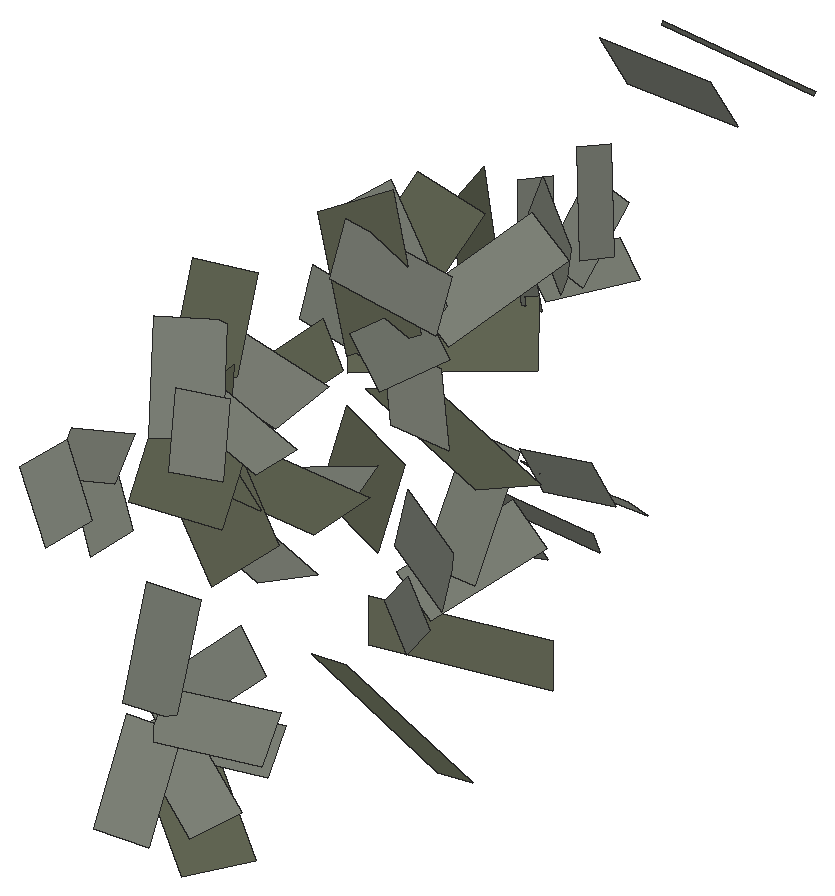
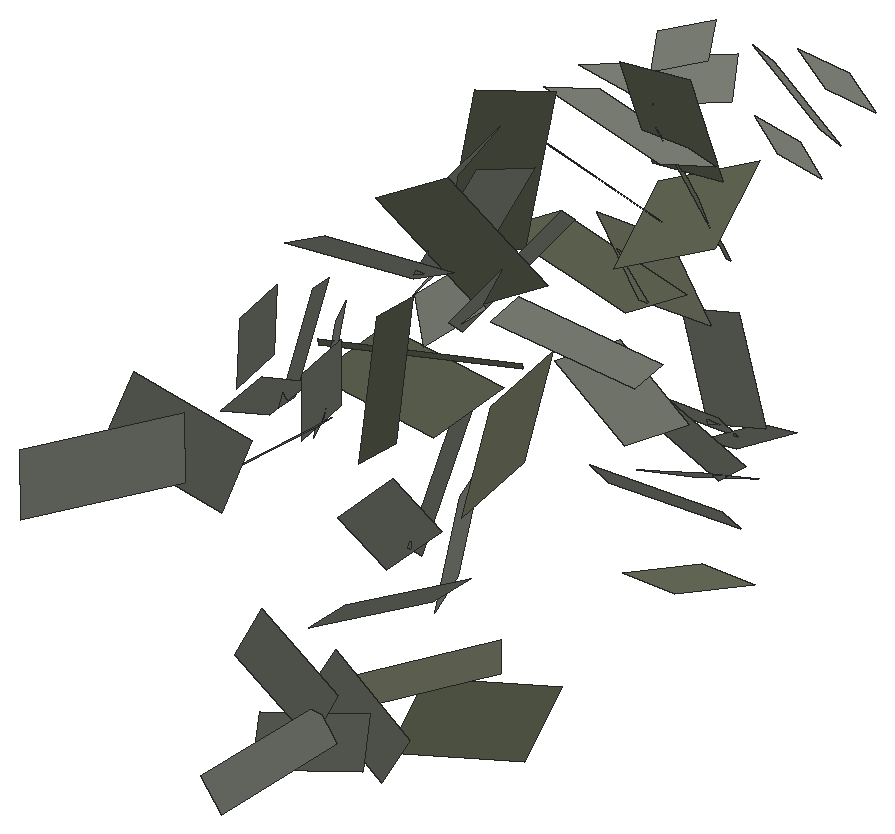
# SketchUp Ruby script. Lengths in inches.
U = 1.inch
M = Sketchup.active_model
def pt(a) = Geom::Point3d.new(a.map { |v| v * U })
def face(e, loops, mat)
  f = e.add_face(loops[0].map { |a| pt(a) })
  loops[1..].each { |l| e.add_face(l.map { |a| pt(a) }).erase! }
  f.material = f.back_material = mat if mat
  f
end
# faces: each face lists its corners as indices into pts; further lists are holes
def faces(e, pts, list, mat = nil) = list.each { |f| face(e, (f[0].is_a?(Array) ? f : [f]).map { |l| l.map { |i| pts[i] } }, mat) }
# xy, xz, yz: faces in a plane at the given z, y or x. An outline is a flat list of corners, or four numbers for a rectangle; further outlines are holes
def ring(l) = l.size == 4 ? [[l[0], l[1]], [l[2], l[1]], [l[2], l[3]], [l[0], l[3]]] : l.each_slice(2).to_a
def flat(e, list, mat, &to3) = list.each { |f| face(e, (f[0].is_a?(Array) ? f : [f]).map { |l| ring(l).map { |u, v| to3.(u, v) } }, mat) }
def xy(e, z, list, mat = nil) = flat(e, list, mat) { |x, y| [x, y, z] }
def xz(e, y, list, mat = nil) = flat(e, list, mat) { |x, z| [x, y, z] }
def yz(e, x, list, mat = nil) = flat(e, list, mat) { |y, z| [x, y, z] }
def lines(e, pts, list) = list.each { |a, b| e.add_line(pt(pts[a]), pt(pts[b])) }
# prism: a flat outline (further loops are holes) pulled along v
def prism(e, loops, v, mat = nil)
  f = face(e, loops, mat); d = Geom::Vector3d.new(v.map { |x| x * U })
  f.pushpull(f.normal.samedirection?(d) ? d.length : -d.length)
end
def box(e, o, s, mat = nil) = prism(e, [[o, [o[0] + s[0], o[1], o[2]], [o[0] + s[0], o[1] + s[1], o[2]], [o[0], o[1] + s[1], o[2]]]], [0, 0, s[2]], mat)
def at(x, y, z, deg = 0) = Geom::Transformation.translation(pt([x, y, z])) * Geom::Transformation.rotation(ORIGIN, Z_AXIS, deg.degrees)
def axes(o, x, y, z) = Geom::Transformation.new([*x, 0, *y, 0, *z, 0, *pt(o).to_a, 1])
def part(name) = M.definitions.add(name)
# library, detail: a bought-in or finely detailed component or shape, given as its bounding box
def library(name, o, s) = part(name).tap { |d| box(d.entities, o, s) }
def detail(e, o, s) = box(e.add_group.entities, o, s)
def put(e, d, t, mat = nil) = e.add_instance(d, t).tap { |i| i.material = mat if mat }
def group(e, t, mat = nil) = e.add_group.tap { |g| g.transformation = t; g.material = mat if mat }.entities
root = M.entities
M.materials.add("viburnumblaasdfas0df1w06d").color = [98, 102, 84]
M.materials.add("viburnumbladsadfasdfad0w122").color = [125, 129, 119]
c1 = part("Component\#314")
p = [[0.14,0,0],[2.58,0.05,0.25],[2.44,5.11,2.64],[0,5.05,2.39]]
faces(c1.entities,p,[[0,1,2,3]],"viburnumblaasdfas0df1w06d")
c2 = part("viburnumblad1\#2")
put(c2.entities,c1,axes([-37.25,6.23,19.31],[75.98784,0,0],[0,65.50676,0],[0,0,75.98784]))
c3 = part("Component\#315")
p = [[0.25,0,0],[2.05,0.01,0.35],[1.81,4.2,1.66],[0,4.19,1.3125]]
faces(c3.entities,p,[[0,1,2,3]],"viburnumbladsadfasdfad0w122")
c4 = part("viburnumblad2")
put(c4.entities,c3,axes([-19.23,-4.49,-32.18],[83.35428,0,0],[0,79.38502,0],[0,0,83.35428]))
put(root,c2,axes([2216.77,275.47,24.61],[-0.00255,0.011,0.00125],[-0.00551,-0.00279,0.01135],[0.00975,0.00148,0.00412]))
put(root,c4,axes([2215.32,257.68,28.24],[0.00143,-0.00635,-0.00868],[0.00992,-0.00012,0.00155],[-0.0013,-0.00861,0.00528]))
put(root,c4,axes([2215.7,277.85,15.48],[-0.00478,-0.00491,0.00751],[0.00915,-0.00588,0.00198],[0.00339,0.00769,0.00718]))
put(root,c2,axes([2216.48,261.41,27.22],[0.01164,0.00293,-0.00079],[-0.00215,0.01041,0.00877],[0.00216,-0.00738,0.00809]))
put(root,c4,axes([2216.16,256.38,28.67],[-0.00668,-0.00514,-0.00687],[0.00865,-0.00485,-0.0047],[-0.00103,-0.00803,0.00606]))
put(root,c4,axes([2216.17,258.49,27.46],[-0.00601,-0.0039,-0.00689],[0.00865,-0.00485,-0.0047],[-0.00175,-0.00854,0.00529]))
put(root,c2,axes([2216.23,265.53,26.16],[-0.01393,-0.0074,0.00333],[0.00558,-0.01491,-0.00981],[0.00654,-0.00631,0.01332]))
put(root,c4,axes([2215.15,286.03,28.11],[-0.00284,-0.00899,0.01128],[0.01228,-0.00546,-0.00125],[0.00539,0.01,0.00933]))
put(root,c2,axes([2215.12,262.56,25.59],[0.00605,-0.00776,-0.00693],[0.01168,0.0029,0.00677],[-0.00267,-0.00844,0.00676]))
put(root,c4,axes([2215.67,279.9375,17.63],[0.0086,-0.00684,0.0012],[0.00538,0.00535,-0.00804],[0.0044,0.00684,0.00749]))
put(root,c4,axes([2215.47,279.03,16.375],[0.00269,-0.008,0.00714],[0.0092,-0.00069,-0.00424],[0.00383,0.00759,0.00707]))
put(root,c4,axes([2215.8,266.32,21.68],[-0.0065,-0.01157,-0.00112],[0.01142,-0.00611,-0.00313],[0.00221,-0.00249,0.0129]))
put(root,c2,axes([2215.51,263.71,15.08],[-0.00788,-0.01001,-0.0014],[0.00865,-0.00529,-0.01087],[0.00682,-0.00657,0.00863]))
put(root,c4,axes([2216.59,258.75,18.54],[0.01026,0.00498,-0.00256],[-0.00015,0.00559,0.01026],[0.0056,-0.00897,0.00496]))
put(root,c4,axes([2218.89,269.98,25.88],[-0.00545,0.00916,0.00529],[-0.00808,-0.00821,0.00589],[0.00818,-0.00089,0.00998]))
put(root,c2,axes([2216.46,272.24,21.13],[-0.00936,-0.00465,0.0096],[0.00338,-0.01554,-0.00424],[0.01026,-0.00044,0.00979]))
put(root,c4,axes([2218.34,276.4,26.26],[-0.00065,0.00993,-0.00423],[-0.00522,0.0028,0.00703],[0.00831,0.00266,0.0042]))
put(root,c4,axes([2215.34,287.43,29.63],[0.00691,-0.01139,0.00621],[0.0117,0.00243,-0.00856],[0.0056,0.00897,0.01021]))
put(root,c2,axes([2214.76,271.4,13.64],[0.00066,-0.01186,0.00699],[0.01121,-0.00532,-0.01007],[0.0098,0.00532,0.0081]))
put(root,c4,axes([2215.58,266.09,23.5],[0.00323,-0.01225,-0.0041],[0.01276,0.00369,-0.00099],[0.00204,-0.00369,0.01263]))
put(root,c2,axes([2216.34,269.37,27.16],[0.01029,0.00428,-0.00658],[0.00078,0.01194,0.00879],[0.00737,-0.00649,0.00685]))
put(root,c4,axes([2217.47,262.76,30.71],[-0.01238,-0.00774,-0.00167],[0.00772,-0.01057,-0.00819],[0.00296,-0.0074,0.01235]))
put(root,c4,axes([2216.15,260.25,18.125],[0.00784,-0.00117,-0.00859],[0.00729,0.00715,0.00568],[0.00468,-0.00917,0.00553]))
put(root,c4,axes([2218.99,269.42,27.52],[0.00288,0.01252,0.00147],[-0.00904,0.00098,0.00938],[0.00888,-0.00309,0.00888]))
put(root,c4,axes([2215.99,261.56,17.28],[0.00079,-0.00637,-0.0092],[0.01172,0.00425,-0.00193],[0.00425,-0.00877,0.00644]))
put(root,c4,axes([2218.42,259.42,17.8],[-0.01026,-0.00498,0.00256],[0.0015,-0.00759,-0.00876],[0.0054,-0.00736,0.0073]))
put(root,c2,axes([2215.96,263.29,26.33],[0.00918,-0.00623,-0.00469],[0.00881,0.01006,0.00379],[0.00131,-0.00544,0.00952]))
put(root,c4,axes([2216.91,279.56,17.11],[-0.0048,-0.00448,0.0089],[0.00915,-0.00588,0.00198],[0.00393,0.00822,0.00626]))
put(root,c2,axes([2215.07,271.54,26.12],[0.00626,-0.00918,-0.00848],[0.01094,0.01129,-0.00412],[0.00772,-0.00395,0.00939]))
put(root,c2,axes([2216.52,264.34,24.43],[-0.00713,-0.00827,-0.00706],[0.01264,-0.00623,-0.00545],[-0.00006,-0.00799,0.0088]))
put(root,c4,axes([2217.31,260.76,17.73],[-0.00667,-0.00821,-0.00496],[0.00888,-0.00228,-0.00816],[0.00454,-0.00802,0.00718]))
put(root,c4,axes([2216.21,264.04,29.79],[-0.0037,-0.01142,-0.00741],[0.01514,-0.00214,-0.00425],[0.00214,-0.0084,0.01187]))
put(root,c4,axes([2217.89,277.41,26.43],[0.00544,-0.00271,-0.00718],[0.0003,0.00981,-0.00339],[0.00825,0.00152,0.00476]))
put(root,c2,axes([2218.31,268.12,27.22],[0.00679,0.01089,0.00142],[-0.00667,0.00218,0.0129],[0.00902,-0.00665,0.00468]))
put(root,c2,axes([2215.76,271.5,16],[0.00753,-0.01126,-0.00255],[0.00884,0.00827,-0.01044],[0.00867,0.00351,0.01012]))
put(root,c4,axes([2218.02,270.95,18.42],[0.00716,-0.00025,-0.0097],[-0.0002,0.01356,-0.00049],[0.01011,0.00042,0.00745]))
put(root,c4,axes([2218.97,276.95,27.07],[0.00435,0.00477,-0.00798],[-0.00392,0.00825,0.00263],[0.00812,0.00193,0.0048]))
put(root,c4,axes([2218.92,276.9,25.2],[-0.0065,0.00265,0.00695],[0.00166,-0.0098,0.00501],[0.00741,0.00415,0.00458]))
put(root,c4,axes([2219.77,276.72,26.18],[-0.00523,0.00868,0.00226],[-0.00357,-0.00459,0.00897],[0.00802,0.00357,0.00411]))
put(root,c2,axes([2216.41,264.9,24.47],[-0.00228,-0.0125,-0.00287],[0.01428,-0.00152,-0.00471],[0.00336,-0.00314,0.01093]))
put(root,c4,axes([2219.37,270.55,19.34],[0.00427,0.00859,-0.00811],[-0.005,0.00913,0.00703],[0.0107,0.00084,0.00653]))
put(root,c4,axes([2220.65,269.3125,28.34],[-0.00501,0.0098,0.00679],[-0.00808,-0.00821,0.00589],[0.00877,-0.00196,0.0093]))
put(root,c4,axes([2217.59,259.75,18.98],[0.00083,-0.00664,-0.00958],[0.01085,0.00394,-0.00179],[0.00425,-0.00877,0.00644]))
put(root,c4,axes([2219.35,270.89,16.85],[-0.00779,-0.00011,0.00854],[0.00262,-0.01208,0.00224],[0.0089,0.00345,0.00816]))
put(root,c4,axes([2220.25,270.54,26.83],[-0.00997,0.00134,0.00814],[-0.00176,-0.01174,-0.00023],[0.00802,-0.0014,0.01005]))
put(root,c4,axes([2220.3125,276.97,27.47],[-0.00062,0.00952,-0.00405],[-0.0058,0.00311,0.00781],[0.00831,0.00266,0.0042]))
put(root,c4,axes([2219.27,271.32,25.85],[-0.00949,-0.00826,0.00492],[0.00532,-0.00908,-0.00498],[0.00706,-0.00173,0.0107]))
put(root,c4,axes([2220.34,270.28,18.08],[-0.00627,0.00896,0.00619],[-0.00305,-0.00837,0.00903],[0.01046,0.00298,0.00629]))
put(root,c4,axes([2219.68,260.23,29.75],[-0.0092,-0.00594,0.0008],[0.00497,-0.0084,-0.00522],[0.00323,-0.00386,0.00866]))
put(root,c2,axes([2217.09,272.57,23.67],[-0.00406,-0.01328,0.00293],[0.01275,-0.00581,-0.00863],[0.008,0.00014,0.01172]))
put(root,c4,axes([2218.53,270.8125,28.3],[0.00997,-0.00134,-0.00814],[0.0038,0.01207,0.00267],[0.00731,-0.00445,0.00969]))
put(root,c4,axes([2218.71,261.17,29.3],[-0.00331,-0.00841,-0.00433],[0.01007,-0.00189,-0.00393],[0.00222,-0.00567,0.00805]))
